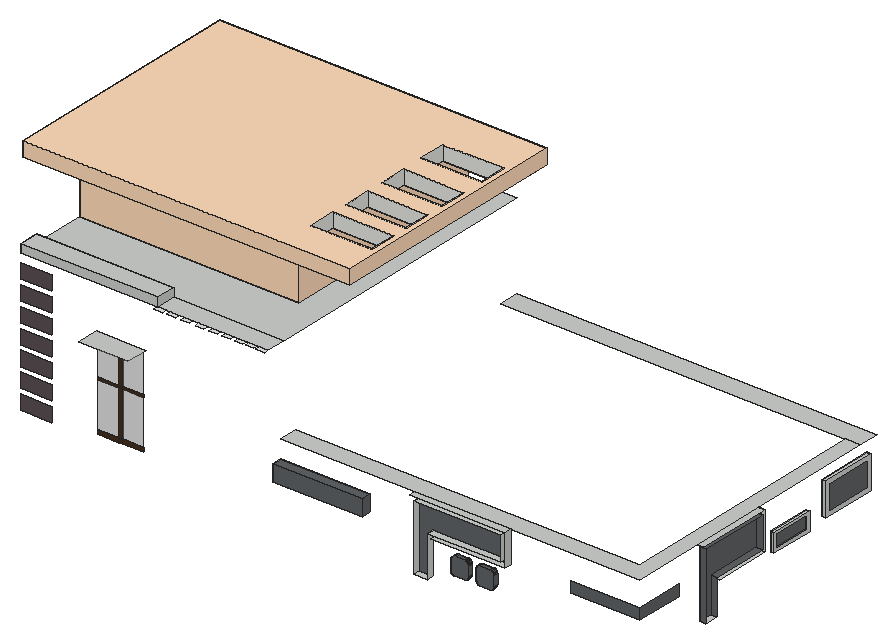
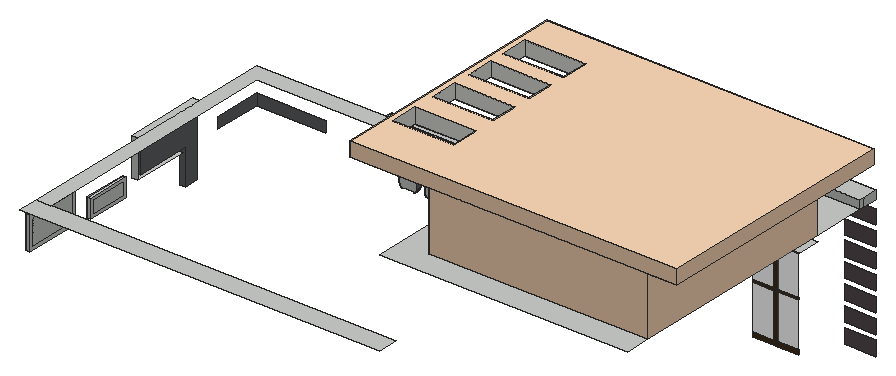
# SketchUp Ruby script. Lengths in inches.
U = 1.inch
M = Sketchup.active_model
def pt(a) = Geom::Point3d.new(a.map { |v| v * U })
def face(e, loops, mat)
  f = e.add_face(loops[0].map { |a| pt(a) })
  loops[1..].each { |l| e.add_face(l.map { |a| pt(a) }).erase! }
  f.material = f.back_material = mat if mat
  f
end
# faces: each face lists its corners as indices into pts; further lists are holes
def faces(e, pts, list, mat = nil) = list.each { |f| face(e, (f[0].is_a?(Array) ? f : [f]).map { |l| l.map { |i| pts[i] } }, mat) }
# xy, xz, yz: faces in a plane at the given z, y or x. An outline is a flat list of corners, or four numbers for a rectangle; further outlines are holes
def ring(l) = l.size == 4 ? [[l[0], l[1]], [l[2], l[1]], [l[2], l[3]], [l[0], l[3]]] : l.each_slice(2).to_a
def flat(e, list, mat, &to3) = list.each { |f| face(e, (f[0].is_a?(Array) ? f : [f]).map { |l| ring(l).map { |u, v| to3.(u, v) } }, mat) }
def xy(e, z, list, mat = nil) = flat(e, list, mat) { |x, y| [x, y, z] }
def xz(e, y, list, mat = nil) = flat(e, list, mat) { |x, z| [x, y, z] }
def yz(e, x, list, mat = nil) = flat(e, list, mat) { |y, z| [x, y, z] }
def lines(e, pts, list) = list.each { |a, b| e.add_line(pt(pts[a]), pt(pts[b])) }
# prism: a flat outline (further loops are holes) pulled along v
def prism(e, loops, v, mat = nil)
  f = face(e, loops, mat); d = Geom::Vector3d.new(v.map { |x| x * U })
  f.pushpull(f.normal.samedirection?(d) ? d.length : -d.length)
end
def box(e, o, s, mat = nil) = prism(e, [[o, [o[0] + s[0], o[1], o[2]], [o[0] + s[0], o[1] + s[1], o[2]], [o[0], o[1] + s[1], o[2]]]], [0, 0, s[2]], mat)
def at(x, y, z, deg = 0) = Geom::Transformation.translation(pt([x, y, z])) * Geom::Transformation.rotation(ORIGIN, Z_AXIS, deg.degrees)
def axes(o, x, y, z) = Geom::Transformation.new([*x, 0, *y, 0, *z, 0, *pt(o).to_a, 1])
def part(name) = M.definitions.add(name)
# library, detail: a bought-in or finely detailed component or shape, given as its bounding box
def library(name, o, s) = part(name).tap { |d| box(d.entities, o, s) }
def detail(e, o, s) = box(e.add_group.entities, o, s)
def put(e, d, t, mat = nil) = e.add_instance(d, t).tap { |i| i.material = mat if mat }
def group(e, t, mat = nil) = e.add_group.tap { |g| g.transformation = t; g.material = mat if mat }.entities
root = M.entities
M.materials.add("[0027_PeachPuff]").color = [255, 218, 185]
M.materials.add("[Asphalt New]").color = [89, 79, 82]
M.materials.add("[Basic Tile]").color = [203, 206, 202]
M.materials.add("[Blacktop Old 01]").color = [96, 99, 102]
M.materials.add("[Polished Concrete Old]").color = [229, 229, 229]
M.materials.add("[Translucent Glass Gray]").color = [128, 128, 128]
M.materials["[Translucent Glass Gray]"].alpha = 0.5
M.materials.add("[Wood Floor]").color = [71, 48, 28]
xy(root,773.48,[[1345.67,861.53,1356.61,885.41]],"[Basic Tile]")
xy(root,774.51,[[958.95,718.33,983.3,730.52]],"[Basic Tile]")
xy(root,793.37,[[1026.3,723.58,1045.02,730.52],[1071.21,723.58,1088.8,730.52]],"[Basic Tile]")
xy(root,814.05,[[1345.67,1016.59,1351.55,1093.89]],"[Basic Tile]")
xy(root,818.75,[[1345.67,1021.29,1348.05,1089.2]],"[Basic Tile]")
xy(root,818.75,[[1348.05,1021.29,1351.55,1089.2]],"[Blacktop Old 01]")
xy(root,821.08,[[1345.67,1128.05,1352.99,1226.23]],"[Basic Tile]")
xy(root,824.81,[[1030.01,723.58,1043.7,730.52],[1071.47,723.58,1088.97,730.52]],"[Blacktop Old 01]")
xy(root,827.26,[[1345.67,1134.23,1352.49,1220.05],[1352.49,1134.23,1352.99,1220.05]],"[Basic Tile]")
xy(root,829.875,[[1345.67,891.02,1356.61,990.33]],"[Basic Tile]")
xy(root,835.48,[[1345.67,885.41,1356.61,984.72]],"[Blacktop Old 01]")
xy(root,836.5625,[[716.67,713.41,873.36,730.52]],"[Blacktop Old 01]")
xy(root,840.25,[[989.93,718.33,1118.75,730.52]],"[Basic Tile]")
xy(root,841.86,[[1345.67,1021.29,1348.05,1089.2]],"[Basic Tile]")
xy(root,841.86,[[1348.05,1021.29,1351.55,1089.2]],"[Blacktop Old 01]")
xy(root,846.55,[[1345.67,1016.59,1351.55,1093.89]],"[Basic Tile]")
xy(root,846.89,[[983.3,718.33,1112.11,730.52]],"[Basic Tile]")
xy(root,864.5625,[[716.67,713.41,873.36,730.52]],"[Blacktop Old 01]")
xy(root,872.39,[[1345.67,1134.23,1352.49,1220.05],[1352.49,1134.23,1352.99,1220.05]],"[Basic Tile]")
xy(root,878.58,[[1345.67,1128.05,1352.99,1226.23]],"[Basic Tile]")
xy(root,889.3,[[958.95,718.33,1112.11,730.52]],"[Basic Tile]")
xy(root,890.33,[[1345.67,861.53,1356.61,984.72]],"[Blacktop Old 01]")
xy(root,895.9375,[[952.31,718.33,1118.75,730.52],[716.67,730.52,1345.67,730.52,1345.67,1212.51,1319.77,1212.51,1319.77,762.76,716.67,762.76],[1345.67,855.93,1356.61,990.33],[716.67,1212.51,1345.67,1247.67]],"[Basic Tile]")
xy(root,943.81,[[385.1,703.09,471.56,741.66]],"[Basic Tile]")
xy(root,1047.125,[[282.77,703.09,523.06,738.33],[523.06,703.09,716.67,738.33],[282.77,738.33,716.67,738.33,716.67,1247.67,282.77,1247.67,282.77,1203.05,666.31,1203.05,666.31,833.98,282.77,833.98],[282.77,833.98,666.31,1203.05]],"[Basic Tile]")
xy(root,1047.125,[[523.06,695.28,537.89,703.09],[545.87,695.28,560.71,703.09],[570.43,695.28,585.27,703.09],[595.93,695.28,610.77,703.09],[619.62,695.28,634.46,703.09],
  [642.37,695.28,657.21,703.09],[664.18,695.28,679.02,703.09],[683.01,695.28,697.85,703.09],[701.84,695.28,716.67,703.09]],"[Polished Concrete Old]")
xy(root,1062.1875,[[282.77,703.09,523.06,738.33]],"[Basic Tile]")
xy(root,1149.875,[[282.77,833.98,666.31,1203.05]])
xy(root,1149.875,[[[231.33,772.48,231.33,1203.05,282.77,1203.05,282.77,833.98,666.31,833.98,666.31,1203.05,804.06,1203.05,804.06,772.48],[687.24,833.67,793.37,882.23],[687.24,908.92,793.37,957.48],[687.24,987.54,793.37,1036.11],[687.24,1074.48,793.37,1123.04]]],"[0027_PeachPuff]")
xy(root,1175.25,[[[231.33,772.48,804.06,1203.05],[687.24,833.67,793.37,882.23],[687.24,908.92,793.37,957.48],[687.24,987.54,793.37,1036.11],[687.24,1074.48,793.37,1123.04]]],"[0027_PeachPuff]")
xz(root,703.09,[[282.77,800.89,338.2,826.14],[282.77,835.2,338.2,860.45],[282.77,869.52,338.2,894.77],[282.77,903.83,338.2,929.08],[282.77,938.14,338.2,963.39],
  [282.77,972.45,338.2,997.7],[282.77,1006.77,338.2,1032.02]],"[Asphalt New]")
xz(root,703.09,[[282.77,1047.125,523.06,1062.1875]],"[Basic Tile]")
xz(root,713.41,[[716.67,836.5625,873.36,864.5625]],"[Blacktop Old 01]")
xz(root,723.58,[[1026.3,793.37,1045.02,793.37,1045.87,793.43,1046.7,793.59,1047.51,793.86,1048.27,794.24,1048.98,794.71,1049.61,795.27,1050.17,795.91,1050.65,796.62,1051.02,797.38,1051.3,798.19,1051.46,799.02,1051.52,799.87,1051.52,816.99,1051.45,818.01,1051.25,819.01,1050.92,819.98,1050.47,820.9,1049.9,821.75,1049.23,822.52,1048.46,823.19,1047.61,823.76,1046.6875,824.21,1045.72,824.54,1044.72,824.74,1043.7,824.81,1030.01,824.81,1028.71,824.72,1027.4375,824.47,1026.21,824.05,1025.04,823.48,1023.96,822.76,1022.99,821.9,1022.13,820.92,1021.41,819.84,1020.83,818.68,1020.42,817.45,1020.16,816.18,1020.08,814.88,1020.08,799.59,1020.13,798.78,1020.29,797.98,1020.55,797.21,1020.91,796.48,1021.36,795.8,1021.9,795.19,1022.51,794.66,1023.1875,794.2,1023.92,793.84,1024.6875,793.58,1025.49,793.42],[1071.21,793.37,1088.8,793.37,1089.74,793.43,1090.65,793.61,1091.54,793.91,1092.38,794.33,1093.16,794.85,1093.86,795.47,1094.48,796.17,1095,796.95,1095.41,797.79,1095.71,798.67,1095.89,799.59,1095.95,800.52,1095.95,817.82,1095.89,818.73,1095.72,819.63,1095.42,820.49,1095.02,821.31,1094.51,822.07,1093.91,822.76,1093.22,823.36,1092.46,823.87,1091.64,824.28,1090.78,824.57,1089.88,824.75,1088.97,824.81,1071.47,824.81,1070.5625,824.75,1069.67,824.57,1068.81,824.28,1067.99,823.875,1067.24,823.37,1066.55,822.77,1065.95,822.09,1065.45,821.33,1065.05,820.51,1064.75,819.65,1064.58,818.76,1064.52,817.85,1064.52,800.07,1064.57,799.19,1064.75,798.33,1065.03,797.5,1065.41,796.72,1065.9,795.99,1066.48,795.33,1067.14,794.75,1067.87,794.27,1068.65,793.88,1069.48,793.6,1070.34,793.43]],"[Blacktop Old 01]")
xz(root,730.52,[[1026.3,793.37,1025.49,793.42,1024.6875,793.58,1023.92,793.84,1023.1875,794.2,1022.51,794.66,1021.9,795.19,1021.36,795.8,1020.91,796.48,1020.55,797.21,1020.29,797.98,1020.13,798.78,1020.08,799.59,1020.08,814.88,1020.16,816.18,1020.42,817.45,1020.83,818.68,1021.41,819.84,1022.13,820.92,1022.99,821.9,1023.96,822.76,1025.04,823.48,1026.21,824.05,1027.4375,824.47,1028.71,824.72,1030.01,824.81,1043.7,824.81,1044.72,824.74,1045.72,824.54,1046.6875,824.21,1047.61,823.76,1048.46,823.19,1049.23,822.52,1049.9,821.75,1050.47,820.9,1050.92,819.98,1051.25,819.01,1051.45,818.01,1051.52,816.99,1051.52,799.87,1051.46,799.02,1051.3,798.19,1051.02,797.38,1050.65,796.62,1050.17,795.91,1049.61,795.27,1048.98,794.71,1048.27,794.24,1047.51,793.86,1046.7,793.59,1045.87,793.43,1045.02,793.37],[1071.21,793.37,1070.34,793.43,1069.48,793.6,1068.65,793.88,1067.87,794.27,1067.14,794.75,1066.48,795.33,1065.9,795.99,1065.41,796.72,1065.03,797.5,1064.75,798.33,1064.57,799.19,1064.52,800.07,1064.52,817.85,1064.58,818.76,1064.75,819.65,1065.05,820.51,1065.45,821.33,1065.95,822.09,1066.55,822.77,1067.24,823.37,1067.99,823.875,1068.81,824.28,1069.67,824.57,1070.5625,824.75,1071.47,824.81,1088.97,824.81,1089.88,824.75,1090.78,824.57,1091.64,824.28,1092.46,823.87,1093.22,823.36,1093.91,822.76,1094.51,822.07,1095.02,821.31,1095.42,820.49,1095.72,819.63,1095.89,818.73,1095.95,817.82,1095.95,800.52,1095.89,799.59,1095.71,798.67,1095.41,797.79,1095,796.95,1094.48,796.17,1093.86,795.47,1093.16,794.85,1092.38,794.33,1091.54,793.91,1090.65,793.61,1089.74,793.43,1088.8,793.37],[716.67,836.5625,873.36,864.5625]],"[Basic Tile]")
xz(root,730.52,[[958.95,774.51,983.3,774.51,983.3,846.89,1112.11,846.89,1112.11,889.3,958.95,889.3],[1224.56,832.66,1345.67,852.16]],"[Blacktop Old 01]")
xz(root,738.33,[[282.77,1047.125,523.06,1062.1875]],"[Basic Tile]")
xz(root,741.66,[[387.85,790.65,425.21,868.86],[430.65,790.65,468.81,868.86],[387.85,872.83,425.21,941.07],[430.65,872.83,468.81,941.07]],"[Translucent Glass Gray]")
xz(root,741.66,[[387.85,783.4,425.21,790.65],[425.21,783.4,430.65,790.65],[430.65,783.4,468.81,790.65],[425.21,790.65,430.65,868.86],[387.85,868.86,425.21,872.83],
  [425.21,868.86,430.65,872.83],[430.65,868.86,468.81,872.83],[425.21,872.83,430.65,941.07]],"[Wood Floor]")
xz(root,772.48,[[231.33,1149.875,804.06,1175.25]],"[0027_PeachPuff]")
xz(root,833.67,[[687.24,1149.875,793.37,1175.25]])
xz(root,833.98,[[282.77,1047.125,666.31,1149.875]],"[0027_PeachPuff]")
xz(root,861.53,[[1345.67,773.48,1356.61,890.33]],"[Blacktop Old 01]")
xz(root,882.23,[[687.24,1149.875,793.37,1175.25]])
xz(root,885.41,[[1345.67,773.48,1356.61,835.48]],"[Blacktop Old 01]")
xz(root,908.92,[[687.24,1149.875,793.37,1175.25]])
xz(root,957.48,[[687.24,1149.875,793.37,1175.25]])
xz(root,984.72,[[1345.67,835.48,1356.61,890.33]],"[Blacktop Old 01]")
xz(root,987.54,[[687.24,1149.875,793.37,1175.25]])
xz(root,990.33,[[1345.67,829.875,1356.61,895.9375]],"[Basic Tile]")
xz(root,1016.59,[[1345.67,814.05,1351.55,846.55]],"[Basic Tile]")
xz(root,1021.29,[[1345.67,818.75,1348.05,841.86]],"[Basic Tile]")
xz(root,1021.29,[[1348.05,818.75,1351.55,841.86]],"[Blacktop Old 01]")
xz(root,1036.11,[[687.24,1149.875,793.37,1175.25]])
xz(root,1074.48,[[687.24,1149.875,793.37,1175.25]])
xz(root,1089.2,[[1345.67,818.75,1348.05,841.86]],"[Basic Tile]")
xz(root,1089.2,[[1348.05,818.75,1351.55,841.86]],"[Blacktop Old 01]")
xz(root,1093.89,[[1345.67,814.05,1351.55,846.55]],"[Basic Tile]")
xz(root,1123.04,[[687.24,1149.875,793.37,1175.25]])
xz(root,1128.05,[[1345.67,821.08,1352.99,878.58]],"[Basic Tile]")
xz(root,1134.23,[[1345.67,827.26,1352.49,872.39],[1352.49,827.26,1352.99,872.39]],"[Basic Tile]")
xz(root,1203.05,[[282.77,1047.125,666.31,1149.875],[231.33,1149.875,804.06,1175.25]],"[0027_PeachPuff]")
xz(root,1220.05,[[1345.67,827.26,1352.49,872.39],[1352.49,827.26,1352.99,872.39]],"[Basic Tile]")
xz(root,1226.23,[[1345.67,821.08,1352.99,878.58]],"[Basic Tile]")
yz(root,231.33,[[772.48,1149.875,1203.05,1175.25]],"[0027_PeachPuff]")
yz(root,282.77,[[833.98,1047.125,1203.05,1149.875]],"[0027_PeachPuff]")
yz(root,282.77,[[703.09,1047.125,730.52,1062.1875],[730.52,1047.125,738.33,1062.1875]],"[Basic Tile]")
yz(root,523.06,[[703.09,1047.125,738.33,1062.1875]],"[Basic Tile]")
yz(root,666.31,[[833.98,1047.125,1203.05,1149.875]],"[0027_PeachPuff]")
yz(root,687.24,[[833.67,1149.875,882.23,1175.25],[908.92,1149.875,957.48,1175.25],[987.54,1149.875,1036.11,1175.25],[1074.48,1149.875,1123.04,1175.25]])
yz(root,716.67,[[713.41,836.5625,730.52,864.5625]],"[Basic Tile]")
yz(root,793.37,[[833.67,1149.875,882.23,1175.25],[908.92,1149.875,957.48,1175.25],[987.54,1149.875,1036.11,1175.25],[1074.48,1149.875,1123.04,1175.25]])
yz(root,804.06,[[772.48,1149.875,1203.05,1175.25]],"[0027_PeachPuff]")
yz(root,873.36,[[713.41,836.5625,730.52,864.5625]],"[Blacktop Old 01]")
yz(root,958.95,[[718.33,774.51,730.52,889.3]],"[Basic Tile]")
yz(root,983.3,[[718.33,774.51,730.52,846.89]],"[Basic Tile]")
yz(root,1020.08,[[723.58,799.59,730.52,814.88]],"[Blacktop Old 01]")
yz(root,1051.52,[[723.58,799.87,730.52,816.99]],"[Blacktop Old 01]")
yz(root,1064.52,[[723.58,800.07,730.52,817.85]],"[Blacktop Old 01]")
yz(root,1095.95,[[723.58,800.52,730.52,817.82]],"[Blacktop Old 01]")
yz(root,1112.11,[[718.33,846.89,730.52,889.3]],"[Basic Tile]")
yz(root,1118.75,[[718.33,840.25,730.52,895.9375]],"[Basic Tile]")
yz(root,1345.67,[[[1016.59,814.05,1093.89,846.55],[1021.29,818.75,1089.2,841.86]],[1021.29,818.75,1089.2,841.86],[[1128.05,821.08,1226.23,878.58],[1134.23,827.26,1220.05,872.39]],[1134.23,827.26,1220.05,872.39]],"[Basic Tile]")
yz(root,1345.67,[[861.53,773.48,885.41,773.48,885.41,835.48,984.72,835.48,984.72,890.33,861.53,890.33],[730.52,832.66,814.64,852.16]],"[Blacktop Old 01]")
yz(root,1348.05,[[1021.29,818.75,1089.2,841.86]],"[Blacktop Old 01]")
yz(root,1351.55,[[[1016.59,814.05,1093.89,846.55],[1021.29,818.75,1089.2,841.86]]],"[Basic Tile]")
yz(root,1352.49,[[1134.23,827.26,1220.05,872.39]],"[Blacktop Old 01]")
yz(root,1352.99,[[[1128.05,821.08,1226.23,878.58],[1134.23,827.26,1220.05,872.39]]],"[Basic Tile]")
p = [[1024.6875,730.52,793.58],[1025.49,730.52,793.42],[1025.49,723.58,793.42],[1024.6875,723.58,793.58],[1026.3,730.52,793.37],[1026.3,723.58,793.37],
  [1045.02,730.52,793.37],[1045.87,730.52,793.43],[1045.87,723.58,793.43],[1045.02,723.58,793.37],[1046.7,730.52,793.59],[1046.7,723.58,793.59],
  [1069.48,730.52,793.6],[1070.34,730.52,793.43],[1070.34,723.58,793.43],[1069.48,723.58,793.6],[1071.21,730.52,793.37],[1071.21,723.58,793.37],
  [1088.8,730.52,793.37],[1089.74,730.52,793.43],[1089.74,723.58,793.43],[1088.8,723.58,793.37],[1090.65,730.52,793.61],[1090.65,723.58,793.61],
  [1023.92,730.52,793.84],[1023.92,723.58,793.84],[1047.51,730.52,793.86],[1047.51,723.58,793.86],[1068.65,730.52,793.88],[1068.65,723.58,793.88],
  [1091.54,730.52,793.91],[1091.54,723.58,793.91],[1023.1875,730.52,794.2],[1023.1875,723.58,794.2],[1048.27,730.52,794.24],[1048.27,723.58,794.24],
  [1067.87,730.52,794.27],[1067.87,723.58,794.27],[1092.38,730.52,794.33],[1092.38,723.58,794.33],[1022.51,730.52,794.66],[1022.51,723.58,794.66],
  [1048.98,730.52,794.71],[1048.98,723.58,794.71],[1067.14,730.52,794.75],[1067.14,723.58,794.75],[1093.16,730.52,794.85],[1093.16,723.58,794.85],
  [1021.9,730.52,795.19],[1021.9,723.58,795.19],[1049.61,730.52,795.27],[1049.61,723.58,795.27],[1066.48,730.52,795.33],[1066.48,723.58,795.33],
  [1093.86,730.52,795.47],[1093.86,723.58,795.47],[1021.36,730.52,795.8],[1021.36,723.58,795.8],[1050.17,730.52,795.91],[1050.17,723.58,795.91],
  [1065.9,730.52,795.99],[1065.9,723.58,795.99],[1094.48,730.52,796.17],[1094.48,723.58,796.17],[1020.91,730.52,796.48],[1020.91,723.58,796.48],
  [1050.65,730.52,796.62],[1050.65,723.58,796.62],[1065.41,730.52,796.72],[1065.41,723.58,796.72],[1095,730.52,796.95],[1095,723.58,796.95],
  [1020.55,730.52,797.21],[1020.55,723.58,797.21],[1051.02,730.52,797.38],[1051.02,723.58,797.38],[1065.03,730.52,797.5],[1065.03,723.58,797.5],
  [1095.41,730.52,797.79],[1095.41,723.58,797.79],[1020.29,730.52,797.98],[1020.29,723.58,797.98],[1051.3,730.52,798.19],[1051.3,723.58,798.19],
  [1064.75,730.52,798.33],[1064.75,723.58,798.33],[1095.71,730.52,798.67],[1095.71,723.58,798.67],[1020.13,730.52,798.78],[1020.13,723.58,798.78],
  [1051.46,730.52,799.02],[1051.46,723.58,799.02],[1064.57,730.52,799.19],[1064.57,723.58,799.19],[1095.89,730.52,799.59],[1095.89,723.58,799.59],
  [1020.08,730.52,799.59],[1020.08,723.58,799.59],[1051.52,730.52,799.87],[1051.52,723.58,799.87],[1064.52,730.52,800.07],[1064.52,723.58,800.07],
  [1095.95,730.52,800.52],[1095.95,723.58,800.52],[1020.16,730.52,816.18],[1020.08,730.52,814.88],[1020.08,723.58,814.88],[1020.16,723.58,816.18],
  [1020.42,730.52,817.45],[1020.42,723.58,817.45],[1051.52,730.52,816.99],[1051.45,730.52,818.01],[1051.45,723.58,818.01],[1051.52,723.58,816.99],
  [1020.83,730.52,818.68],[1020.83,723.58,818.68],[1095.95,730.52,817.82],[1095.89,730.52,818.73],[1095.89,723.58,818.73],[1095.95,723.58,817.82],
  [1064.58,730.52,818.76],[1064.52,730.52,817.85],[1064.52,723.58,817.85],[1064.58,723.58,818.76],[1051.25,730.52,819.01],[1051.25,723.58,819.01],
  [1021.41,730.52,819.84],[1021.41,723.58,819.84],[1095.72,730.52,819.63],[1095.72,723.58,819.63],[1064.75,730.52,819.65],[1064.75,723.58,819.65],
  [1050.92,730.52,819.98],[1050.92,723.58,819.98],[1095.42,730.52,820.49],[1095.42,723.58,820.49],[1065.05,730.52,820.51],[1065.05,723.58,820.51],
  [1022.13,730.52,820.92],[1022.13,723.58,820.92],[1050.47,730.52,820.9],[1050.47,723.58,820.9],[1065.45,730.52,821.33],[1065.45,723.58,821.33],
  [1095.02,730.52,821.31],[1095.02,723.58,821.31],[1022.99,730.52,821.9],[1022.99,723.58,821.9],[1049.9,730.52,821.75],[1049.9,723.58,821.75],
  [1065.95,730.52,822.09],[1065.95,723.58,822.09],[1094.51,730.52,822.07],[1094.51,723.58,822.07],[1049.23,730.52,822.52],[1049.23,723.58,822.52],
  [1023.96,730.52,822.76],[1023.96,723.58,822.76],[1066.55,730.52,822.77],[1066.55,723.58,822.77],[1093.91,730.52,822.76],[1093.91,723.58,822.76],
  [1048.46,730.52,823.19],[1048.46,723.58,823.19],[1025.04,730.52,823.48],[1025.04,723.58,823.48],[1067.24,730.52,823.37],[1067.24,723.58,823.37],
  [1093.22,730.52,823.36],[1093.22,723.58,823.36],[1047.61,730.52,823.76],[1047.61,723.58,823.76],[1067.99,730.52,823.875],[1067.99,723.58,823.875],
  [1092.46,730.52,823.87],[1092.46,723.58,823.87],[1026.21,730.52,824.05],[1026.21,723.58,824.05],[1046.6875,730.52,824.21],[1046.6875,723.58,824.21],
  [1068.81,730.52,824.28],[1068.81,723.58,824.28],[1091.64,730.52,824.28],[1091.64,723.58,824.28],[1027.4375,730.52,824.47],[1027.4375,723.58,824.47],
  [1045.72,730.52,824.54],[1045.72,723.58,824.54],[1069.67,730.52,824.57],[1069.67,723.58,824.57],[1090.78,730.52,824.57],[1090.78,723.58,824.57],
  [1028.71,730.52,824.72],[1028.71,723.58,824.72],[1044.72,730.52,824.74],[1044.72,723.58,824.74],[1070.5625,730.52,824.75],[1070.5625,723.58,824.75],
  [1089.88,730.52,824.75],[1089.88,723.58,824.75],[1030.01,730.52,824.81],[1030.01,723.58,824.81],[1043.7,730.52,824.81],[1043.7,723.58,824.81],
  [1071.47,730.52,824.81],[1071.47,723.58,824.81],[1088.97,730.52,824.81],[1088.97,723.58,824.81]]
faces(root,p,[[0,1,2,3],[1,4,5,2],[6,7,8,9],[7,10,11,8],[12,13,14,15],[13,16,17,14],[18,19,20,21],[19,22,23,20],
  [24,0,3,25],[10,26,27,11],[28,12,15,29],[22,30,31,23],[32,24,25,33],[26,34,35,27],[36,28,29,37],[30,38,39,31],
  [40,32,33,41],[34,42,43,35],[44,36,37,45],[38,46,47,39],[48,40,41,49],[42,50,51,43],[52,44,45,53],[46,54,55,47],
  [56,48,49,57],[50,58,59,51],[60,52,53,61],[54,62,63,55],[64,56,57,65],[58,66,67,59],[68,60,61,69],[62,70,71,63],
  [72,64,65,73],[66,74,75,67],[76,68,69,77],[70,78,79,71],[80,72,73,81],[74,82,83,75],[84,76,77,85],[78,86,87,79],
  [88,80,81,89],[82,90,91,83],[92,84,85,93],[86,94,95,87],[96,88,89,97],[90,98,99,91],[100,92,93,101],[94,102,103,95],
  [104,105,106,107],[108,104,107,109],[110,111,112,113],[114,108,109,115],[116,117,118,119],[120,121,122,123],[111,124,125,112],[126,114,115,127],
  [117,128,129,118],[130,120,123,131],[124,132,133,125],[128,134,135,129],[136,130,131,137],[138,126,127,139],[132,140,141,133],[142,136,137,143],
  [134,144,145,135],[146,138,139,147],[140,148,149,141],[150,142,143,151],[144,152,153,145],[148,154,155,149],[156,146,147,157],[158,150,151,159],
  [152,160,161,153],[154,162,163,155],[164,156,157,165],[166,158,159,167],[160,168,169,161],[162,170,171,163],[172,166,167,173],[168,174,175,169],
  [176,164,165,177],[170,178,179,171],[180,172,173,181],[174,182,183,175],[184,176,177,185],[178,186,187,179],[188,180,181,189],[182,190,191,183],
  [192,184,185,193],[186,194,195,187],[196,188,189,197],[190,198,199,191],[200,192,193,201],[194,202,203,195],[204,196,197,205],[198,206,207,199]],"[Blacktop Old 01]")
